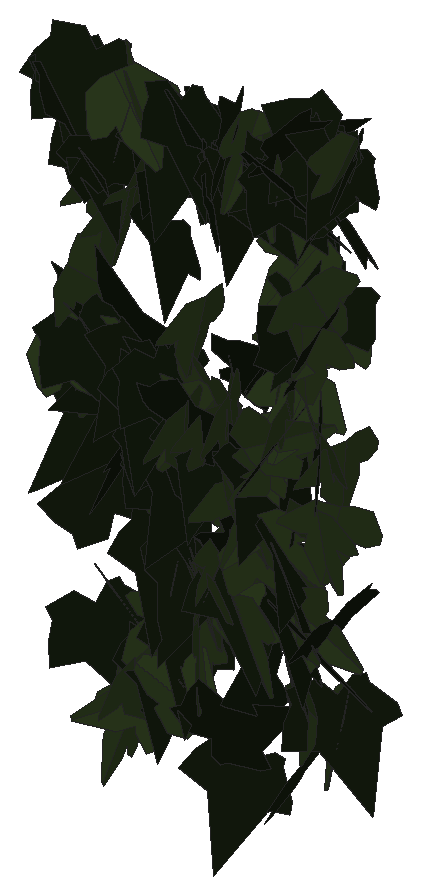
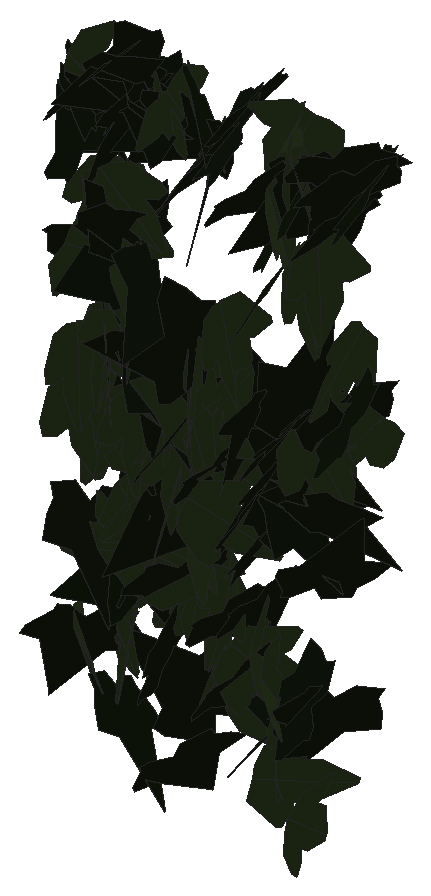
# SketchUp Ruby script. Lengths in inches.
U = 1.inch
M = Sketchup.active_model
def pt(a) = Geom::Point3d.new(a.map { |v| v * U })
def face(e, loops, mat)
  f = e.add_face(loops[0].map { |a| pt(a) })
  loops[1..].each { |l| e.add_face(l.map { |a| pt(a) }).erase! }
  f.material = f.back_material = mat if mat
  f
end
# faces: each face lists its corners as indices into pts; further lists are holes
def faces(e, pts, list, mat = nil) = list.each { |f| face(e, (f[0].is_a?(Array) ? f : [f]).map { |l| l.map { |i| pts[i] } }, mat) }
# xy, xz, yz: faces in a plane at the given z, y or x. An outline is a flat list of corners, or four numbers for a rectangle; further outlines are holes
def ring(l) = l.size == 4 ? [[l[0], l[1]], [l[2], l[1]], [l[2], l[3]], [l[0], l[3]]] : l.each_slice(2).to_a
def flat(e, list, mat, &to3) = list.each { |f| face(e, (f[0].is_a?(Array) ? f : [f]).map { |l| ring(l).map { |u, v| to3.(u, v) } }, mat) }
def xy(e, z, list, mat = nil) = flat(e, list, mat) { |x, y| [x, y, z] }
def xz(e, y, list, mat = nil) = flat(e, list, mat) { |x, z| [x, y, z] }
def yz(e, x, list, mat = nil) = flat(e, list, mat) { |y, z| [x, y, z] }
def lines(e, pts, list) = list.each { |a, b| e.add_line(pt(pts[a]), pt(pts[b])) }
# prism: a flat outline (further loops are holes) pulled along v
def prism(e, loops, v, mat = nil)
  f = face(e, loops, mat); d = Geom::Vector3d.new(v.map { |x| x * U })
  f.pushpull(f.normal.samedirection?(d) ? d.length : -d.length)
end
def box(e, o, s, mat = nil) = prism(e, [[o, [o[0] + s[0], o[1], o[2]], [o[0] + s[0], o[1] + s[1], o[2]], [o[0], o[1] + s[1], o[2]]]], [0, 0, s[2]], mat)
def at(x, y, z, deg = 0) = Geom::Transformation.translation(pt([x, y, z])) * Geom::Transformation.rotation(ORIGIN, Z_AXIS, deg.degrees)
def axes(o, x, y, z) = Geom::Transformation.new([*x, 0, *y, 0, *z, 0, *pt(o).to_a, 1])
def part(name) = M.definitions.add(name)
# library, detail: a bought-in or finely detailed component or shape, given as its bounding box
def library(name, o, s) = part(name).tap { |d| box(d.entities, o, s) }
def detail(e, o, s) = box(e.add_group.entities, o, s)
def put(e, d, t, mat = nil) = e.add_instance(d, t).tap { |i| i.material = mat if mat }
def group(e, t, mat = nil) = e.add_group.tap { |g| g.transformation = t; g.material = mat if mat }.entities
root = M.entities
M.materials.add("efeu1").color = [18, 25, 13]
M.materials.add("efeu2").color = [43, 57, 29]
c1 = part("ivyleaf_10")
p = [[0,0.5,-0.03],[-0.0625,2.02,-0.43],[-0.19,2.01,-0.46],[-0.54,1.05,-0.29],[-0.52,0.625,-0.18],[-0.83,0.76,-0.28],
  [-1.16,0.64,-0.33],[-1.15,0.33,-0.24],[-0.77,-0.39,0.02],[-0.3,-0.51,0.16],[0.04,-0.48,0.23],[-0.02,2.01,-0.4375],
  [-0.06,2.01,-0.43],[0.04,-0.49,0.23],[0.67,-0.49,0.14],[1.38,0.36,-0.2],[1.375,0.51,-0.24],[0.81,0.65,-0.19],
  [0.62,0.59,-0.15],[0.6,1.09,-0.28],[0.5,1.23,-0.31]]
faces(c1.entities,p,[[0,1,2,3,4,5,6,7,8,9,10],[11,12,0,13,14,15,16,17,18,19,20]],"efeu2")
c2 = part("ivyleaf_9")
p = [[1.54,2.16,1.25],[1.36,2.04,1.19],[-0.21,0.99,0.68],[-0.71,1.11,0.82],[-0.85,0.86,0.67],[-0.8,0.17,0.21],
  [-0.9,-0.01,0.1],[-0.67,-0.16,-0.02],[-0.08,-0.08,-0.05],[-0.03,-0.6,-0.4],[0.65,-0.88,-0.66],[0.83,-0.6,-0.49],
  [1.29,-0.42,-0.43],[1.8125,-0.07,-0.26],[1.21,0.44,0.15]]
faces(c2.entities,p,[[0,1,2,3,4,5,6,7,8,9,10,11,12,13,14]],"efeu1")
put(root,c1,axes([23.44,223.3,218.89],[0.00637,-0.48208,-0.13251],[-0.00395,0.13246,-0.48212],[0.49994,0.00719,-0.00213]))
put(root,c2,axes([24.8,223.67,216.28],[0.10403,-0.35819,0.33299],[0.11817,-0.31194,-0.37247],[0.47457,0.15619,0.01975]))
put(root,c2,axes([22.66,223.68,218.79],[-0.01558,-0.46816,0.17489],[0.01548,-0.17535,-0.46799],[0.49952,-0.00916,0.01996]))
put(root,c1,axes([25.29,223.33,220.58],[-0.47244,-0.15841,0.04135],[-0.03815,-0.01628,-0.49828],[0.15921,-0.47396,0.0033]))
put(root,c2,axes([23.89,223.35,214.64],[0.01623,-0.07422,0.49419],[0.47666,-0.14623,-0.03761],[0.15011,0.47234,0.06601]))
put(root,c2,axes([23.25,223.53,222.98],[0.11977,-0.48434,-0.03267],[-0.00646,0.03205,-0.49893],[0.4854,0.11994,0.00142]))
put(root,c1,axes([25.72,223.42,218.22],[-0.37871,-0.30879,0.10598],[-0.07881,-0.07104,-0.48861],[0.31681,-0.38679,0.00513]))
put(root,c2,axes([23.13,223.77,217.61],[-0.06155,-0.3943,0.30123],[-0.04256,-0.29822,-0.39906],[0.49437,-0.07477,0.00315]))
put(root,c2,axes([23.18,223.4,218.6875],[0.2163,-0.09564,0.44053],[0.40655,-0.16973,-0.23646],[0.19477,0.46049,0.00434]))
put(root,c1,axes([23.46,223.4,214.91],[0.18265,0.13852,0.44436],[-0.43505,-0.11887,0.21588],[0.16545,-0.46549,0.0771]))
put(root,c1,axes([25.42,223.33,218.11],[-0.48548,0.09718,-0.06976],[0.07043,-0.00349,-0.495],[-0.09669,-0.49045,-0.0103]))
put(root,c1,axes([24.47,223.64,218],[0.12537,0.32891,-0.35511],[-0.14128,-0.32599,-0.35181],[-0.46295,0.18855,0.0112]))
put(root,c2,axes([24.8,223.74,216.78],[0.04938,-0.21502,0.4487],[0.13841,-0.42717,-0.21993],[0.47792,0.14593,0.01734]))
put(root,c2,axes([23.92,223.76,221.98],[0.04397,-0.43688,0.23917],[0.01813,-0.23854,-0.43906],[0.49773,0.04729,-0.00513]))
put(root,c2,axes([21.8,223.39,219.51],[0.08295,-0.39125,-0.30007],[-0.00344,0.30382,-0.39709],[0.49306,0.06794,0.04771]))
put(root,c1,axes([22.46,223.36,222.94],[0.36721,0.21876,0.25943],[0.22467,0.12975,-0.42742],[-0.25432,0.43048,-0.00301]))
put(root,c2,axes([24.8,223.375,218.94],[-0.24974,0.42039,-0.10442],[0.04954,-0.09202,-0.48896],[-0.43032,-0.25457,0.00431]))
put(root,c2,axes([25.59,223.22,219.32],[0.04652,-0.03064,-0.49689],[-0.47686,0.14058,-0.05331],[0.14297,0.47885,-0.01614]))
put(root,c1,axes([24.1,223.33,219.28],[0.09617,-0.44058,-0.21596],[0.00063,0.22018,-0.44891],[0.49066,0.08607,0.0429]))
put(root,c1,axes([24.79,223.64,219.95],[0.12548,-0.42037,-0.23988],[0.09847,-0.22046,0.43784],[-0.47388,-0.15712,0.02746]))
put(root,c2,axes([24.27,223.8125,218.17],[-0.02166,-0.4284,0.25691],[0.00456,-0.25731,-0.42868],[0.49951,-0.01622,0.01505]))
put(root,c1,axes([24.21,223.51,216.34],[-0.37352,0.22208,-0.24731],[0.18991,-0.16272,-0.43296],[-0.27279,-0.41737,0.03721]))
put(root,c2,axes([21.37,223.59,222.55],[0.27862,-0.4124,0.04799],[0.02608,-0.0403,-0.49769],[0.41436,0.27983,-0.00095]))
put(root,c2,axes([22.43,223.86,219.04],[-0.15646,-0.38935,0.2719],[-0.01816,-0.28116,-0.41306],[0.47454,-0.13913,0.07384]))
put(root,c1,axes([25.38,223.35,221.21],[-0.23876,-0.38011,-0.22025],[0.11886,0.18544,-0.44887],[0.42293,-0.2667,0.00181]))
put(root,c2,axes([24.0625,223.48,222.51],[-0.08214,-0.19756,-0.45191],[0.35005,0.29938,-0.19451],[0.34744,-0.34834,0.08913]))
put(root,c1,axes([24.39,223.61,222.63],[0.37208,-0.16239,0.29187],[0.28423,-0.07551,-0.40436],[0.17541,0.46683,0.03612]))
put(root,c1,axes([24.58,223.39,218.82],[-0.16803,-0.21881,0.417],[0.36132,0.22405,0.26316],[-0.30202,0.38977,0.08283]))
put(root,c2,axes([24.49,223.42,222.54],[0.4724,-0.12229,0.10904],[0.10813,-0.01728,-0.48786],[0.12309,0.48451,0.01012]))
put(root,c1,axes([23.72,223.74,217.05],[0.12802,-0.41601,0.24606],[0.08591,-0.23091,-0.43509],[0.47564,0.15367,0.01235]))
put(root,c1,axes([24.2,223.48,218.07],[-0.22689,-0.43869,-0.0779],[0.05303,0.06021,-0.49352],[0.44239,-0.23222,0.0192]))
put(root,c2,axes([24.07,223.8,214.14],[-0.18334,-0.4626,0.04882],[-0.00909,-0.04891,-0.49752],[0.46508,-0.18332,0.00952]))
put(root,c1,axes([23.04,223.77,215.8],[-0.20046,-0.26942,0.37044],[-0.15832,-0.33869,-0.332],[0.42983,-0.2504,0.05048]))
put(root,c2,axes([25.16,223.32,220.36],[-0.15324,-0.19286,0.43512],[0.32478,0.29177,0.2437],[-0.3479,0.35732,0.03585]))
put(root,c2,axes([24.7,223.89,217.3],[0.04539,-0.39417,0.30425],[0.01247,-0.30451,-0.39638],[0.49778,0.04357,-0.01782]))
put(root,c1,axes([23.44,223.6875,215.78],[-0.09792,0.38869,-0.29889],[0.08027,-0.28797,-0.40079],[-0.4837,-0.12647,-0.006]))
put(root,c1,axes([21.55,223.35,219.21],[0.23765,0.28599,0.33426],[0.21039,0.25977,-0.37183],[-0.38634,0.31738,0.00313]))
put(root,c1,axes([22.59,223.4375,215.07],[-0.01523,-0.45714,-0.20197],[0.04082,0.20025,-0.45633],[0.4981,-0.03039,0.03122]))
put(root,c1,axes([24.57,223.43,217.63],[-0.38391,-0.08677,-0.30836],[0.29658,0.08562,-0.39333],[0.12106,-0.48491,-0.01427]))
put(root,c1,axes([24.2,223.71,222.85],[0.07512,0.41081,-0.27494],[-0.09386,-0.26118,-0.4159],[-0.48533,0.1141,0.03787]))
put(root,c2,axes([22.8,223.83,216.71],[-0.05516,-0.4926,0.06557],[-0.00574,-0.06534,-0.49568],[0.49691,-0.05544,0.00156]))
put(root,c1,axes([25.46,223.4,219.25],[-0.40825,0.21745,0.18987],[-0.16419,0.09557,-0.4625],[-0.23743,-0.43998,-0.00663]))
put(root,c1,axes([25.45,223.84,222.91],[0.06592,-0.38366,0.31378],[0.09617,-0.30063,-0.38778],[0.48622,0.11148,0.03415]))
put(root,c2,axes([22.16,223.3125,222.24],[-0.01016,-0.05319,-0.49706],[0.12455,0.48121,-0.05404],[0.48413,-0.12491,0.00347]))
put(root,c2,axes([21.74,223.7,222.1],[0.10684,-0.48142,-0.08259],[-0.0184,0.08052,-0.49313],[0.48811,0.10841,-0.00051]))
put(root,c2,axes([23.77,223.38,222.25],[0.25436,-0.12246,-0.41268],[-0.37221,0.17822,-0.2823],[0.21623,0.45082,-0.0005]))
put(root,c1,axes([24.91,223.42,219.47],[0.08088,-0.40795,-0.27755],[-0.01987,0.27833,-0.4149],[0.49301,0.07815,0.02881]))
put(root,c1,axes([23.61,223.49,216.64],[-0.42637,0.25801,0.04046],[-0.03821,0.015,-0.49831],[-0.25835,-0.42803,0.00693]))
put(root,c1,axes([24.62,223.74,216.49],[0.06537,-0.10499,0.48446],[0.47862,-0.11383,-0.08925],[0.12904,0.47541,0.08562]))
put(root,c2,axes([22.35,223.96,218.42],[0.00629,-0.03178,-0.49895],[0.13698,-0.47979,0.03229],[-0.48083,-0.13709,0.00267]))
put(root,c1,axes([24.38,223.45,217.38],[-0.22012,-0.22384,-0.38915],[0.36402,0.16467,-0.30062],[0.26275,-0.41566,0.09047]))
put(root,c2,axes([22.63,223.91,214.96],[0.02892,-0.45942,0.19518],[0.05735,-0.19116,-0.45844],[0.49586,0.0489,0.04164]))
put(root,c2,axes([22.12,223.59,217.03],[-0.36094,-0.32587,0.1163],[0.08556,0.07879,0.48628],[-0.33526,0.37094,-0.00112]))
put(root,c1,axes([23.61,223.7,218.73],[0.01724,-0.49689,0.05298],[-0.00341,-0.05313,-0.49716],[0.49969,0.01678,-0.00522]))
put(root,c2,axes([24.79,223.61,216.375],[0.42407,-0.22216,0.14425],[0.13093,-0.0609,-0.47869],[0.23026,0.44378,0.00653]))
put(root,c2,axes([24.26,224.01,215.32],[-0.03638,-0.17916,0.46538],[-0.10983,-0.45228,-0.1827],[0.48643,-0.11552,-0.00644]))
put(root,c2,axes([22.55,223.74,218.94],[-0.00745,-0.02284,-0.49942],[-0.3533,-0.35315,0.02142],[-0.35372,0.35321,-0.01088]))
put(root,c1,axes([23.41,223.82,218.79],[-0.23603,-0.32537,0.29736],[-0.12609,-0.27337,-0.39921],[0.42236,-0.26344,0.047]))
put(root,c1,axes([22.48,223.54,218.77],[-0.33297,-0.00697,-0.37294],[0.37241,0.02201,-0.33291],[0.02106,-0.49947,-0.00946]))
put(root,c2,axes([21.65,223.85,222.97],[-0.25,-0.42455,-0.08518],[0.07558,0.05406,-0.49129],[0.42637,-0.25852,0.03715]))
put(root,c2,axes([25.62,223.45,216.79],[-0.08739,0.49081,-0.03835],[0.00823,-0.03749,-0.49852],[-0.49224,-0.08776,-0.00153]))
put(root,c1,axes([25.65,223.62,219.02],[-0.12316,-0.48038,-0.06377],[0.00645,0.06417,-0.49582],[0.48455,-0.12296,-0.00961]))
put(root,c1,axes([25.01,223.63,216.5],[0.13445,-0.00648,0.48154],[0.47734,0.06805,-0.13236],[-0.06383,0.4953,0.02448]))
put(root,c2,axes([22.71,223.54,218.38],[0.25079,-0.33609,-0.27229],[-0.10034,0.26096,-0.41452],[0.42075,0.26257,0.06345]))
put(root,c1,axes([21.72,223.39,220.26],[0.0119,-0.34118,-0.36531],[0.12934,0.35507,-0.32741],[0.48284,-0.08671,0.0967]))
put(root,c1,axes([25.26,223.4,215.42],[0.10614,-0.08326,-0.48146],[-0.30783,0.37121,-0.13206],[0.37944,0.32445,0.02754]))
put(root,c2,axes([24.0625,223.35,222.74],[-0.22364,0.11356,-0.43254],[-0.40169,0.16154,0.2501],[0.19654,0.45936,0.01898]))
put(root,c2,axes([24.72,223.53,222.63],[0.1472,-0.33224,-0.34344],[-0.10437,0.32833,-0.36236],[0.4663,0.17837,0.02731]))
put(root,c1,axes([24,223.625,216.35],[-0.03395,-0.08661,-0.49127],[0.49799,-0.03476,-0.02828],[-0.02926,-0.49121,0.08862]))
put(root,c2,axes([22.46,223.72,218.2],[-0.25318,0.33536,-0.27098],[0.15711,-0.22088,-0.42015],[-0.40152,-0.2979,0.00647]))
put(root,c1,axes([22.52,223.91,214.47],[0.08289,0.07646,-0.48712],[-0.37947,-0.30552,-0.11252],[-0.31486,0.38834,0.00738]))
put(root,c2,axes([23.37,223.96,218.34],[-0.0848,-0.48267,0.0992],[-0.00889,-0.09915,-0.48999],[0.49268,-0.08487,0.00823]))
put(root,c1,axes([24.17,223.34,217.9],[-0.08817,0.19052,-0.45379],[-0.18578,0.41403,0.20992],[0.45575,0.20563,-0.00222]))
put(root,c2,axes([21.95,223.88,218.23],[-0.4698,-0.1646,0.04685],[-0.04199,-0.02183,-0.49776],[0.16591,-0.47162,0.00669]))
put(root,c2,axes([21.88,223.625,215.58],[-0.03073,-0.36532,-0.34],[0.05728,0.33581,-0.36599],[0.49576,-0.06144,0.02121]))
put(root,c2,axes([25.09,223.54,214.5],[-0.25515,0.42999,-0.00178],[0.00004,-0.00204,-0.5],[-0.43,-0.25515,0.00101]))
put(root,c1,axes([24.92,223.72,219.58],[0.46812,0.12459,-0.12386],[-0.12072,-0.028,-0.4844],[-0.12764,0.48342,0.00386]))
put(root,c1,axes([23.38,223.72,220.14],[-0.01297,-0.4998,0.00568],[0.00027,-0.00569,-0.49997],[0.49983,-0.01297,0.00042]))
put(root,c2,axes([22.35,224.04,221.8],[0.0471,-0.32144,0.38008],[0.07107,-0.37352,-0.3247],[0.49268,0.08461,0.01051]))
put(root,c1,axes([22,223.85,219.07],[-0.23782,-0.38061,0.2204],[-0.08601,-0.20547,-0.44764],[0.43133,-0.25083,0.03226]))
put(root,c2,axes([23.07,223.96,215.62],[-0.00834,-0.49532,0.06774],[-0.0028,-0.0677,-0.49539],[0.49992,-0.00865,-0.00164]))
put(root,c1,axes([22.6875,224,216.09],[0.05909,-0.13687,0.47726],[0.33569,-0.3431,-0.13996],[0.36581,0.33697,0.05135]))
put(root,c2,axes([22.78,223.62,219.24],[0.08873,-0.36816,-0.32647],[-0.08742,0.31466,-0.37861],[0.48424,0.12427,-0.00853]))
put(root,c2,axes([24.08,223.39,217.48],[0.40733,0.25716,0.13398],[0.10593,0.0831,-0.48153],[-0.26993,0.42067,0.01322]))
put(root,c2,axes([25.13,223.98,222.93],[-0.4022,-0.23173,0.18583],[-0.15984,-0.09481,-0.46418],[0.25037,-0.43279,0.00219]))
put(root,c2,axes([23.99,223.84,216.69],[-0.12147,-0.45381,-0.17117],[0.0685,0.15864,-0.46919],[0.48016,-0.13743,0.02364]))
put(root,c2,axes([23.96,223.66,219.57],[0.36481,-0.08509,0.33117],[0.31676,-0.09825,-0.37418],[0.12875,0.48281,-0.01778]))
put(root,c1,axes([22.18,223.76,221.2],[-0.00046,-0.5,-0.00211],[-0.00057,0.00211,-0.5],[0.5,-0.00046,-0.00058]))
put(root,c2,axes([23.14,224.03,216.5],[-0.18259,-0.45515,0.09749],[-0.02287,-0.09582,-0.4902],[0.46491,-0.18347,0.01417]))
put(root,c1,axes([22.03,224.05,214.07],[-0.01662,-0.28263,0.41212],[0.2177,-0.37526,-0.24857],[0.44981,0.17117,0.13553]))
put(root,c1,axes([25.01,223.77,221.47],[0.42948,0.01753,-0.25541],[-0.25542,-0.00476,-0.42981],[-0.0175,0.49967,0.00486]))
put(root,c2,axes([23.16,223.77,222.8125],[0.35321,-0.35354,-0.01607],[-0.01048,0.01224,-0.49974],[0.35375,0.35336,0.00123]))
put(root,c2,axes([21.39,223.92,219.53],[0.24999,-0.38713,0.19399],[0.11026,-0.1597,-0.4608],[0.41874,0.27317,0.00553]))
put(root,c1,axes([24.3125,223.75,218.72],[-0.40324,-0.11091,-0.27404],[0.29342,-0.09352,-0.3939],[0.03612,-0.47849,0.14051]))
put(root,c2,axes([25.28,224.02,221.96],[0.06313,-0.29933,0.3955],[0.21757,-0.34157,-0.29324],[0.44573,0.20913,0.08712]))
put(root,c1,axes([22.22,223.85,222.67],[0.3053,-0.39108,0.06201],[0.03437,-0.05184,-0.49612],[0.39447,0.30719,-0.00477]))
put(root,c1,axes([22.55,223.83,222.01],[0.19671,-0.45872,0.02966],[0.01601,-0.0254,-0.4991],[0.4594,0.19731,0.00469]))
put(root,c2,axes([22.8125,224.04,222.24],[-0.10367,-0.48014,0.09337],[0.01105,-0.09772,-0.49023],[0.48901,-0.09958,0.03087]))
put(root,c1,axes([25.38,224.02,220.625],[0.1188,0.25673,-0.41228],[-0.1574,-0.38117,-0.28272],[-0.45947,0.19696,-0.00975]))
put(root,c1,axes([23.4,223.67,216.5],[-0.44729,0.22306,-0.01306],[0.01228,-0.00464,-0.49983],[-0.22311,-0.44746,-0.00132]))
put(root,c1,axes([24.26,223.64,217.61],[-0.30964,0.39135,0.03119],[-0.01983,0.02408,-0.49903],[-0.39208,-0.31027,0.00061]))
put(root,c2,axes([25.53,223.87,222.78],[-0.35603,0.22885,-0.26622],[0.21484,-0.15786,-0.423],[-0.27765,-0.41558,0.01407]))
put(root,c2,axes([21.43,223.79,222.79],[0.05429,-0.43838,-0.23425],[0.03371,0.23835,-0.43824],[0.4959,0.03179,0.05544]))
put(root,c1,axes([25.34,223.94,215.33],[0.33738,-0.29397,0.22306],[0.16106,-0.15463,-0.44738],[0.33202,0.37372,-0.00964]))
put(root,c2,axes([25.28,224.04,220.91],[-0.36129,-0.33936,0.06559],[-0.04935,-0.04326,-0.49567],[0.3421,-0.36464,-0.00223]))
put(root,c2,axes([25.26,224.13,222.78],[-0.11851,-0.42309,0.23865],[0.01749,-0.2492,-0.43312],[0.48544,-0.09431,0.07387]))
put(root,c1,axes([24.43,223.85,216.4375],[-0.46504,-0.07503,-0.16767],[-0.16373,-0.03757,0.47093],[-0.08326,0.49291,0.01038]))
put(root,c2,axes([25.43,223.79,215.49],[-0.12762,-0.36679,-0.31493],[0.1276,0.28861,-0.38785],[0.46629,-0.17937,0.01994]))
put(root,c2,axes([22.6,223.85,217.71],[0.19119,-0.45137,-0.09856],[-0.01916,0.09883,-0.48976],[0.46161,0.19105,0.02049]))
put(root,c2,axes([24.78,223.35,222.89],[-0.032,0.28649,-0.40853],[-0.0934,0.3987,0.28691],[0.49016,0.09467,0.028]))
put(root,c2,axes([25.33,223.9,222.51],[-0.40043,0.02767,0.29814],[-0.29834,0.00546,-0.4012],[-0.02546,-0.4992,0.01214]))
put(root,c1,axes([22.64,223.52,222.6],[-0.12109,0.24507,-0.41866],[-0.24401,0.34218,0.27087],[0.41928,0.26992,0.03673]))
put(root,c2,axes([24.67,223.38,220.04],[0.02144,0.37315,0.33211],[0.02225,0.33137,-0.37376],[-0.49904,0.03081,-0.0024]))
put(root,c2,axes([25.22,223.36,220.16],[0.11964,0.19342,0.44528],[0.12349,0.4314,-0.22056],[-0.46951,0.16275,0.05546]))
put(root,c2,axes([24.93,223.57,217.91],[0.0316,-0.01646,0.49873],[-0.2253,0.44542,0.02898],[-0.44525,-0.22655,0.02073]))
put(root,c2,axes([21.99,223.93,215.6],[0.3155,-0.30241,0.24292],[0.16888,-0.1748,-0.43695],[0.3492,0.35777,-0.00816]))
put(root,c2,axes([22.59,224.12,220.85],[0.07517,-0.42996,0.24389],[0.02697,-0.24276,-0.43628],[0.49358,0.07874,-0.0133]))
put(root,c1,axes([22.46,224.06,215.77],[0.21704,-0.28289,0.35052],[0.23036,-0.26464,-0.35623],[0.38707,0.31612,0.01546]))
put(root,c1,axes([21.93,223.79,221.53],[-0.11133,-0.48307,-0.06516],[0.00496,0.06572,-0.49564],[0.48742,-0.11101,-0.00984]))
put(root,c1,axes([23.89,223.62,219.43],[0.25301,-0.31835,-0.29093],[-0.04487,0.31604,-0.38485],[0.42892,0.22085,0.13136]))
put(root,c2,axes([23.47,224.09,222.4],[0.04225,-0.47878,0.13777],[0.00804,-0.13759,-0.48063],[0.49815,0.04283,-0.00392]))
put(root,c1,axes([23.47,223.99,217.7],[-0.19956,-0.0916,0.44921],[-0.34512,-0.29248,-0.21296],[0.30178,-0.39505,0.05351]))
put(root,c2,axes([22.18,223.93,219.34],[0.38201,-0.21173,0.24339],[-0.19357,0.15133,0.43546],[-0.25807,-0.42693,0.03364]))
put(root,c1,axes([23.55,223.79,218.81],[-0.39727,0.11235,-0.28205],[-0.27127,0.07724,0.41285],[0.13633,0.48105,-0.00042]))
put(root,c1,axes([24.52,223.79,218.6],[-0.33342,-0.3703,-0.04133],[0.02886,0.02964,-0.49829],[0.37148,-0.33466,0.00161]))
put(root,c1,axes([24.85,223.67,215.66],[-0.33495,0.34531,0.13626],[-0.11028,0.08268,-0.48063],[-0.35447,-0.35203,0.02077]))
